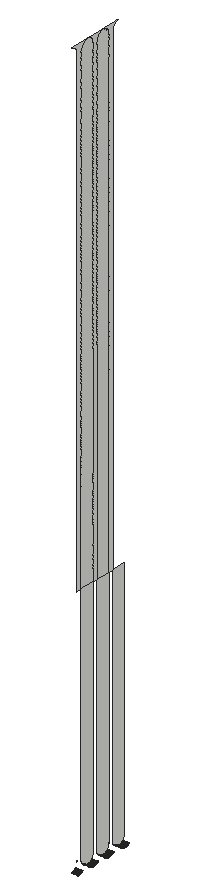
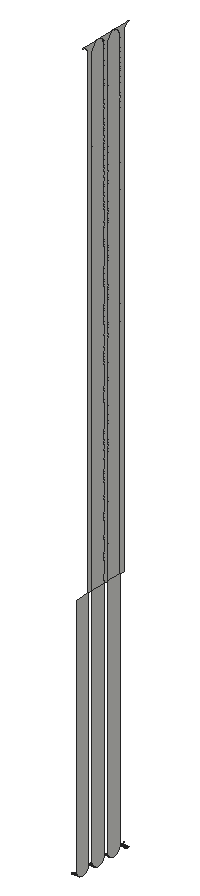
# SketchUp Ruby script. Lengths in inches.
U = 1.inch
M = Sketchup.active_model
def pt(a) = Geom::Point3d.new(a.map { |v| v * U })
def face(e, loops, mat)
  f = e.add_face(loops[0].map { |a| pt(a) })
  loops[1..].each { |l| e.add_face(l.map { |a| pt(a) }).erase! }
  f.material = f.back_material = mat if mat
  f
end
# faces: each face lists its corners as indices into pts; further lists are holes
def faces(e, pts, list, mat = nil) = list.each { |f| face(e, (f[0].is_a?(Array) ? f : [f]).map { |l| l.map { |i| pts[i] } }, mat) }
# xy, xz, yz: faces in a plane at the given z, y or x. An outline is a flat list of corners, or four numbers for a rectangle; further outlines are holes
def ring(l) = l.size == 4 ? [[l[0], l[1]], [l[2], l[1]], [l[2], l[3]], [l[0], l[3]]] : l.each_slice(2).to_a
def flat(e, list, mat, &to3) = list.each { |f| face(e, (f[0].is_a?(Array) ? f : [f]).map { |l| ring(l).map { |u, v| to3.(u, v) } }, mat) }
def xy(e, z, list, mat = nil) = flat(e, list, mat) { |x, y| [x, y, z] }
def xz(e, y, list, mat = nil) = flat(e, list, mat) { |x, z| [x, y, z] }
def yz(e, x, list, mat = nil) = flat(e, list, mat) { |y, z| [x, y, z] }
def lines(e, pts, list) = list.each { |a, b| e.add_line(pt(pts[a]), pt(pts[b])) }
# prism: a flat outline (further loops are holes) pulled along v
def prism(e, loops, v, mat = nil)
  f = face(e, loops, mat); d = Geom::Vector3d.new(v.map { |x| x * U })
  f.pushpull(f.normal.samedirection?(d) ? d.length : -d.length)
end
def box(e, o, s, mat = nil) = prism(e, [[o, [o[0] + s[0], o[1], o[2]], [o[0] + s[0], o[1] + s[1], o[2]], [o[0], o[1] + s[1], o[2]]]], [0, 0, s[2]], mat)
def at(x, y, z, deg = 0) = Geom::Transformation.translation(pt([x, y, z])) * Geom::Transformation.rotation(ORIGIN, Z_AXIS, deg.degrees)
def axes(o, x, y, z) = Geom::Transformation.new([*x, 0, *y, 0, *z, 0, *pt(o).to_a, 1])
def part(name) = M.definitions.add(name)
# library, detail: a bought-in or finely detailed component or shape, given as its bounding box
def library(name, o, s) = part(name).tap { |d| box(d.entities, o, s) }
def detail(e, o, s) = box(e.add_group.entities, o, s)
def put(e, d, t, mat = nil) = e.add_instance(d, t).tap { |i| i.material = mat if mat }
def group(e, t, mat = nil) = e.add_group.tap { |g| g.transformation = t; g.material = mat if mat }.entities
root = M.entities
yz(root,9,[[35.784,2.396,35.842,2.398,35.899,2.403,35.956,2.41,36.012,2.421,36.067,2.435,36.122,2.452,36.176,2.473,36.229,2.495,36.28,2.521,36.329,2.55,36.378,2.581,36.424,2.615,36.468,2.651,36.51,2.69,36.551,2.731,36.588,2.774,36.624,2.82,36.656,2.867,36.687,2.915,36.714,2.966,36.739,3.018,36.761,3.071,36.779,3.125,36.795,3.18,36.808,3.236,36.818,3.292,36.825,3.363,36.825,38,34.743,38,34.743,3.363,34.751,3.292,34.761,3.236,34.773,3.18,34.789,3.125,34.808,3.071,34.83,3.018,34.854,2.966,34.882,2.915,34.912,2.867,34.945,2.82,34.98,2.774,35.018,2.731,35.058,2.69,35.1,2.651,35.145,2.615,35.191,2.581,35.239,2.55,35.289,2.521,35.34,2.495,35.393,2.473,35.446,2.452,35.501,2.435,35.557,2.421,35.613,2.41,35.67,2.403,35.727,2.398],[38.572,2.396,38.629,2.398,38.686,2.403,38.743,2.41,38.799,2.421,38.855,2.435,38.91,2.452,38.963,2.473,39.016,2.495,39.067,2.521,39.117,2.55,39.165,2.581,39.211,2.615,39.256,2.651,39.298,2.69,39.338,2.731,39.376,2.774,39.411,2.82,39.444,2.867,39.474,2.915,39.502,2.966,39.526,3.018,39.548,3.071,39.567,3.125,39.583,3.18,39.595,3.236,39.605,3.292,39.612,3.363,39.612,38,37.531,38,37.531,3.363,37.538,3.292,37.548,3.236,37.561,3.18,37.577,3.125,37.595,3.071,37.617,3.018,37.642,2.966,37.669,2.915,37.7,2.867,37.732,2.82,37.768,2.774,37.805,2.731,37.846,2.69,37.888,2.651,37.932,2.615,37.978,2.581,38.027,2.55,38.076,2.521,38.127,2.495,38.18,2.473,38.234,2.452,38.289,2.435,38.344,2.421,38.4,2.41,38.457,2.403,38.514,2.398],[41.359,2.396,41.417,2.398,41.474,2.403,41.531,2.41,41.587,2.421,41.642,2.435,41.697,2.452,41.751,2.473,41.804,2.495,41.855,2.521,41.904,2.55,41.953,2.581,41.999,2.615,42.043,2.651,42.085,2.69,42.126,2.731,42.163,2.774,42.199,2.82,42.231,2.867,42.262,2.915,42.289,2.966,42.314,3.018,42.336,3.071,42.354,3.125,42.37,3.18,42.383,3.236,42.393,3.292,42.4,3.363,42.4,38,40.318,38,40.318,3.363,40.326,3.292,40.336,3.236,40.348,3.18,40.364,3.125,40.383,3.071,40.405,3.018,40.429,2.966,40.457,2.915,40.487,2.867,40.52,2.82,40.555,2.774,40.593,2.731,40.633,2.69,40.675,2.651,40.72,2.615,40.766,2.581,40.814,2.55,40.864,2.521,40.915,2.495,40.968,2.473,41.021,2.452,41.076,2.435,41.132,2.421,41.188,2.41,41.245,2.403,41.302,2.398],[34.037,3.363,34.04,3.407,34.04,3.464,34.037,3.521],[34.743,3.363,34.743,3.521,34.741,3.464,34.741,3.407],
  [36.825,3.363,36.828,3.407,36.828,3.464,36.825,3.521],[37.531,3.363,37.531,3.521,37.528,3.464,37.528,3.407],[39.612,3.363,39.615,3.407,39.615,3.464,39.612,3.521],[40.318,3.363,40.318,3.521,40.316,3.464,40.316,3.407],[34.037,38,34.743,38,34.743,106.961,34.745,107.015,34.749,107.069,34.756,107.123,34.766,107.177,34.779,107.23,34.794,107.282,34.8125,107.334,34.833,107.384,34.857,107.433,34.883,107.481,34.911,107.528,34.942,107.572,34.975,107.616,35.011,107.657,35.048,107.697,35.088,107.734,35.129,107.769,35.173,107.803,35.217,107.834,35.264,107.862,35.312,107.888,35.361,107.911,35.411,107.932,35.463,107.95,35.515,107.966,35.568,107.979,35.621,107.989,35.675,107.996,35.73,108,33.051,108,33.106,107.996,33.16,107.989,33.213,107.979,33.266,107.966,33.318,107.95,33.37,107.932,33.42,107.911,33.469,107.888,33.517,107.862,33.564,107.834,33.608,107.803,33.652,107.769,33.693,107.734,33.733,107.697,33.77,107.657,33.806,107.616,33.839,107.572,33.87,107.528,33.898,107.481,33.924,107.433,33.948,107.384,33.968,107.334,33.987,107.282,34.002,107.23,34.015,107.177,34.025,107.123,34.032,107.069,34.036,107.015,34.037,106.961],
  [34.743,38,36.825,38,36.825,106.961,36.824,107.015,36.819,107.069,36.812,107.123,36.802,107.177,36.79,107.23,36.774,107.282,36.756,107.334,36.735,107.384,36.712,107.433,36.686,107.481,36.657,107.528,36.626,107.572,36.593,107.616,36.558,107.657,36.52,107.697,36.481,107.734,36.439,107.769,36.396,107.803,36.351,107.834,36.305,107.862,36.257,107.888,36.208,107.911,36.157,107.932,36.106,107.95,36.054,107.966,36.001,107.979,35.947,107.989,35.893,107.996,35.839,108,35.73,108,35.675,107.996,35.621,107.989,35.568,107.979,35.515,107.966,35.463,107.95,35.411,107.932,35.361,107.911,35.312,107.888,35.264,107.862,35.217,107.834,35.173,107.803,35.129,107.769,35.088,107.734,35.048,107.697,35.011,107.657,34.975,107.616,34.942,107.572,34.911,107.528,34.883,107.481,34.857,107.433,34.833,107.384,34.8125,107.334,34.794,107.282,34.779,107.23,34.766,107.177,34.756,107.123,34.749,107.069,34.745,107.015,34.743,106.961],[36.825,38,37.531,38,37.531,106.961,37.532,107.015,37.537,107.069,37.544,107.123,37.554,107.177,37.566,107.23,37.582,107.282,37.6,107.334,37.621,107.384,37.644,107.433,37.67,107.481,37.699,107.528,37.73,107.572,37.763,107.616,37.798,107.657,37.836,107.697,37.875,107.734,37.917,107.769,37.96,107.803,38.005,107.834,38.051,107.862,38.099,107.888,38.148,107.911,38.199,107.932,38.25,107.95,38.302,107.966,38.355,107.979,38.409,107.989,38.463,107.996,38.517,108,35.839,108,35.893,107.996,35.947,107.989,36.001,107.979,36.054,107.966,36.106,107.95,36.157,107.932,36.208,107.911,36.257,107.888,36.305,107.862,36.351,107.834,36.396,107.803,36.439,107.769,36.481,107.734,36.52,107.697,36.558,107.657,36.593,107.616,36.626,107.572,36.657,107.528,36.686,107.481,36.712,107.433,36.735,107.384,36.756,107.334,36.774,107.282,36.79,107.23,36.802,107.177,36.812,107.123,36.819,107.069,36.824,107.015,36.825,106.961],[37.531,38,39.612,38,39.612,106.961,39.611,107.015,39.607,107.069,39.6,107.123,39.59,107.177,39.577,107.23,39.562,107.282,39.543,107.334,39.523,107.384,39.499,107.433,39.473,107.481,39.445,107.528,39.414,107.572,39.381,107.616,39.345,107.657,39.308,107.697,39.268,107.734,39.227,107.769,39.183,107.803,39.139,107.834,39.092,107.862,39.044,107.888,38.995,107.911,38.945,107.932,38.893,107.95,38.841,107.966,38.788,107.979,38.735,107.989,38.681,107.996,38.626,108,38.517,108,38.463,107.996,38.409,107.989,38.355,107.979,38.302,107.966,38.25,107.95,38.199,107.932,38.148,107.911,38.099,107.888,38.051,107.862,38.005,107.834,37.96,107.803,37.917,107.769,37.875,107.734,37.836,107.697,37.798,107.657,37.763,107.616,37.73,107.572,37.699,107.528,37.67,107.481,37.644,107.433,37.621,107.384,37.6,107.334,37.582,107.282,37.566,107.23,37.554,107.177,37.544,107.123,37.537,107.069,37.532,107.015,37.531,106.961],[39.612,38,40.318,38,40.318,106.961,40.32,107.015,40.324,107.069,40.331,107.123,40.341,107.177,40.354,107.23,40.369,107.282,40.388,107.334,40.408,107.384,40.432,107.433,40.458,107.481,40.486,107.528,40.517,107.572,40.55,107.616,40.586,107.657,40.623,107.697,40.663,107.734,40.704,107.769,40.748,107.803,40.792,107.834,40.839,107.862,40.887,107.888,40.936,107.911,40.986,107.932,41.038,107.95,41.09,107.966,41.143,107.979,41.196,107.989,41.25,107.996,41.305,108,38.626,108,38.681,107.996,38.735,107.989,38.788,107.979,38.841,107.966,38.893,107.95,38.945,107.932,38.995,107.911,39.044,107.888,39.092,107.862,39.139,107.834,39.183,107.803,39.227,107.769,39.268,107.734,39.308,107.697,39.345,107.657,39.381,107.616,39.414,107.572,39.445,107.528,39.473,107.481,39.499,107.433,39.523,107.384,39.543,107.334,39.562,107.282,39.577,107.23,39.59,107.177,39.6,107.123,39.607,107.069,39.611,107.015,39.612,106.961]])
p = [[9,33.054,2.398],[9,33.111,2.403],[10,33.111,2.403],[10,33.054,2.398],[9,33.168,2.41],[10,33.168,2.41],
  [9,33.224,2.421],[10,33.224,2.421],[9,33.28,2.435],[10,33.28,2.435],[9,33.335,2.452],[10,33.335,2.452],
  [9,35.446,2.452],[9,35.501,2.435],[10,35.501,2.435],[10,35.446,2.452],[9,35.557,2.421],[10,35.557,2.421],
  [9,35.613,2.41],[10,35.613,2.41],[9,35.67,2.403],[10,35.67,2.403],[9,35.727,2.398],[10,35.727,2.398],
  [9,35.784,2.396],[10,35.784,2.396],[9,35.842,2.398],[10,35.842,2.398],[9,35.899,2.403],[10,35.899,2.403],
  [9,35.956,2.41],[10,35.956,2.41],[9,36.012,2.421],[10,36.012,2.421],[9,36.067,2.435],[10,36.067,2.435],
  [9,36.122,2.452],[10,36.122,2.452],[9,38.234,2.452],[9,38.289,2.435],[10,38.289,2.435],[10,38.234,2.452],
  [9,38.344,2.421],[10,38.344,2.421],[9,38.4,2.41],[10,38.4,2.41],[9,38.457,2.403],[10,38.457,2.403],
  [9,38.514,2.398],[10,38.514,2.398],[9,38.572,2.396],[10,38.572,2.396],[9,38.629,2.398],[10,38.629,2.398],
  [9,38.686,2.403],[10,38.686,2.403],[9,38.743,2.41],[10,38.743,2.41],[9,38.799,2.421],[10,38.799,2.421],
  [9,38.855,2.435],[10,38.855,2.435],[9,38.91,2.452],[10,38.91,2.452],[9,41.021,2.452],[9,41.076,2.435],
  [10,41.076,2.435],[10,41.021,2.452],[9,41.132,2.421],[10,41.132,2.421],[9,41.188,2.41],[10,41.188,2.41],
  [9,41.245,2.403],[10,41.245,2.403],[9,41.302,2.398],[10,41.302,2.398],[9,41.359,2.396],[10,41.359,2.396],
  [9,41.417,2.398],[10,41.417,2.398],[9,41.474,2.403],[10,41.474,2.403],[9,41.531,2.41],[10,41.531,2.41],
  [9,41.587,2.421],[10,41.587,2.421],[9,41.642,2.435],[10,41.642,2.435],[9,41.697,2.452],[10,41.697,2.452],
  [9,33.388,2.473],[10,33.388,2.473],[9,33.441,2.495],[10,33.441,2.495],[9,33.492,2.521],[10,33.492,2.521],
  [9,33.542,2.55],[10,33.542,2.55],[9,33.59,2.581],[10,33.59,2.581],[9,35.191,2.581],[9,35.239,2.55],
  [10,35.239,2.55],[10,35.191,2.581],[9,35.289,2.521],[10,35.289,2.521],[9,35.34,2.495],[10,35.34,2.495],
  [9,35.393,2.473],[10,35.393,2.473],[9,36.176,2.473],[10,36.176,2.473],[9,36.229,2.495],[10,36.229,2.495],
  [9,36.28,2.521],[10,36.28,2.521],[9,36.329,2.55],[10,36.329,2.55],[9,36.378,2.581],[10,36.378,2.581],
  [9,37.978,2.581],[9,38.027,2.55],[10,38.027,2.55],[10,37.978,2.581],[9,38.076,2.521],[10,38.076,2.521],
  [9,38.127,2.495],[10,38.127,2.495],[9,38.18,2.473],[10,38.18,2.473],[9,38.963,2.473],[10,38.963,2.473],
  [9,39.016,2.495],[10,39.016,2.495],[9,39.067,2.521],[10,39.067,2.521],[9,39.117,2.55],[10,39.117,2.55],
  [9,39.165,2.581],[10,39.165,2.581],[9,40.766,2.581],[9,40.814,2.55],[10,40.814,2.55],[10,40.766,2.581],
  [9,40.864,2.521],[10,40.864,2.521],[9,40.915,2.495],[10,40.915,2.495],[9,40.968,2.473],[10,40.968,2.473],
  [9,41.751,2.473],[10,41.751,2.473],[9,41.804,2.495],[10,41.804,2.495],[9,41.855,2.521],[10,41.855,2.521],
  [9,41.904,2.55],[10,41.904,2.55],[9,41.953,2.581],[10,41.953,2.581],[9,33.636,2.615],[10,33.636,2.615],
  [9,33.681,2.651],[10,33.681,2.651],[9,35.1,2.651],[9,35.145,2.615],[10,35.145,2.615],[10,35.1,2.651],
  [9,36.424,2.615],[10,36.424,2.615],[9,36.468,2.651],[10,36.468,2.651],[9,37.888,2.651],[9,37.932,2.615],
  [10,37.932,2.615],[10,37.888,2.651],[9,39.211,2.615],[10,39.211,2.615],[9,39.256,2.651],[10,39.256,2.651],
  [9,40.675,2.651],[9,40.72,2.615],[10,40.72,2.615],[10,40.675,2.651],[9,41.999,2.615],[10,41.999,2.615],
  [9,42.043,2.651],[10,42.043,2.651],[9,33.723,2.69],[10,33.723,2.69],[9,33.763,2.731],[10,33.763,2.731],
  [9,35.058,2.69],[10,35.058,2.69],[9,36.51,2.69],[10,36.51,2.69],[9,36.551,2.731],[10,36.551,2.731],
  [9,37.846,2.69],[10,37.846,2.69],[9,39.298,2.69],[10,39.298,2.69],[9,39.338,2.731],[10,39.338,2.731],
  [9,40.633,2.69],[10,40.633,2.69]]
faces(root,p,[[0,1,2,3],[1,4,5,2],[4,6,7,5],[6,8,9,7],[8,10,11,9],[12,13,14,15],[13,16,17,14],[16,18,19,17],
  [18,20,21,19],[20,22,23,21],[22,24,25,23],[24,26,27,25],[26,28,29,27],[28,30,31,29],[30,32,33,31],[32,34,35,33],
  [34,36,37,35],[38,39,40,41],[39,42,43,40],[42,44,45,43],[44,46,47,45],[46,48,49,47],[48,50,51,49],[50,52,53,51],
  [52,54,55,53],[54,56,57,55],[56,58,59,57],[58,60,61,59],[60,62,63,61],[64,65,66,67],[65,68,69,66],[68,70,71,69],
  [70,72,73,71],[72,74,75,73],[74,76,77,75],[76,78,79,77],[78,80,81,79],[80,82,83,81],[82,84,85,83],[84,86,87,85],
  [86,88,89,87],[10,90,91,11],[90,92,93,91],[92,94,95,93],[94,96,97,95],[96,98,99,97],[100,101,102,103],[101,104,105,102],
  [104,106,107,105],[106,108,109,107],[108,12,15,109],[36,110,111,37],[110,112,113,111],[112,114,115,113],[114,116,117,115],[116,118,119,117],
  [120,121,122,123],[121,124,125,122],[124,126,127,125],[126,128,129,127],[128,38,41,129],[62,130,131,63],[130,132,133,131],[132,134,135,133],
  [134,136,137,135],[136,138,139,137],[140,141,142,143],[141,144,145,142],[144,146,147,145],[146,148,149,147],[148,64,67,149],[88,150,151,89],
  [150,152,153,151],[152,154,155,153],[154,156,157,155],[156,158,159,157],[98,160,161,99],[160,162,163,161],[164,165,166,167],[165,100,103,166],
  [118,168,169,119],[168,170,171,169],[172,173,174,175],[173,120,123,174],[138,176,177,139],[176,178,179,177],[180,181,182,183],[181,140,143,182],
  [158,184,185,159],[184,186,187,185],[162,188,189,163],[188,190,191,189],[192,164,167,193],[170,194,195,171],[194,196,197,195],[198,172,175,199],
  [178,200,201,179],[200,202,203,201],[204,180,183,205]])
